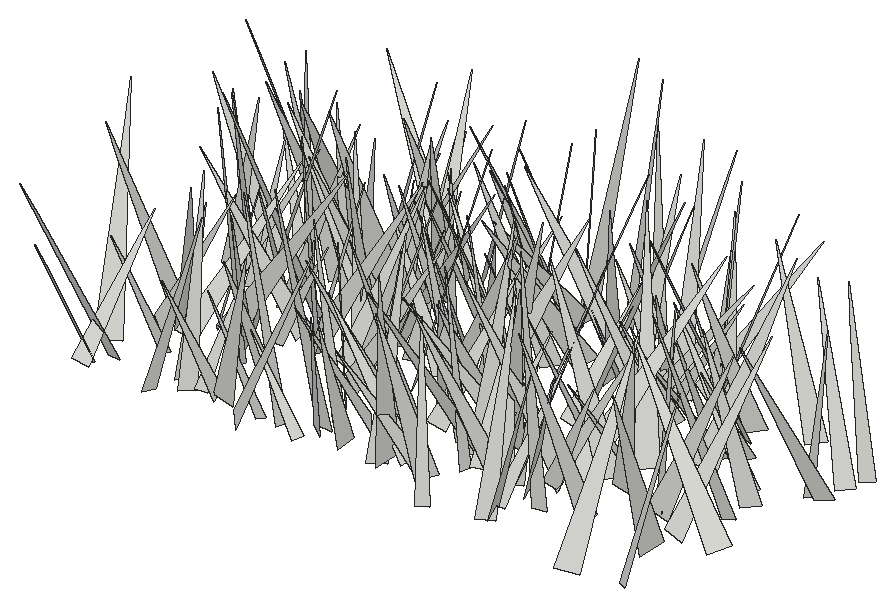
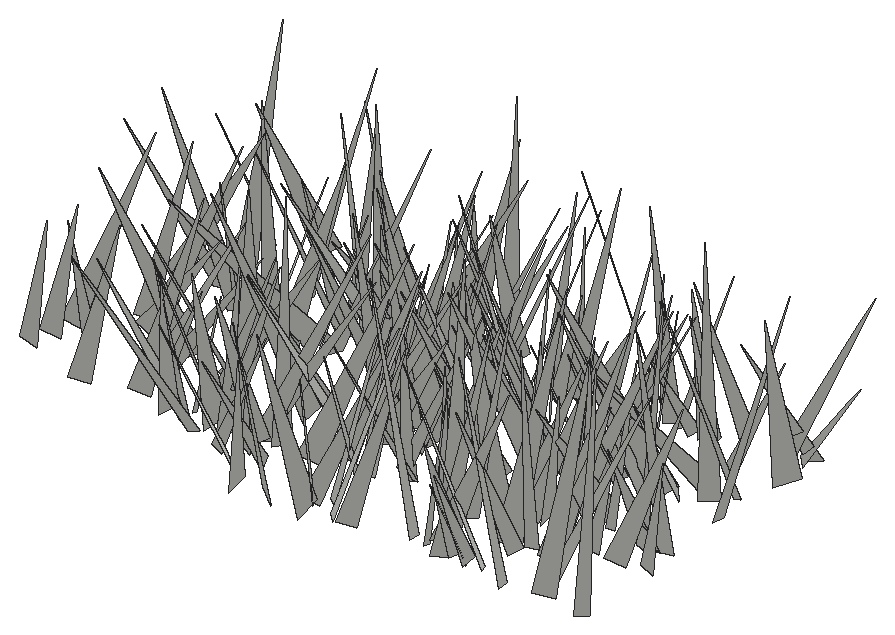
# SketchUp Ruby script. Lengths in inches.
U = 1.inch
M = Sketchup.active_model
def pt(a) = Geom::Point3d.new(a.map { |v| v * U })
def face(e, loops, mat)
  f = e.add_face(loops[0].map { |a| pt(a) })
  loops[1..].each { |l| e.add_face(l.map { |a| pt(a) }).erase! }
  f.material = f.back_material = mat if mat
  f
end
# faces: each face lists its corners as indices into pts; further lists are holes
def faces(e, pts, list, mat = nil) = list.each { |f| face(e, (f[0].is_a?(Array) ? f : [f]).map { |l| l.map { |i| pts[i] } }, mat) }
# xy, xz, yz: faces in a plane at the given z, y or x. An outline is a flat list of corners, or four numbers for a rectangle; further outlines are holes
def ring(l) = l.size == 4 ? [[l[0], l[1]], [l[2], l[1]], [l[2], l[3]], [l[0], l[3]]] : l.each_slice(2).to_a
def flat(e, list, mat, &to3) = list.each { |f| face(e, (f[0].is_a?(Array) ? f : [f]).map { |l| ring(l).map { |u, v| to3.(u, v) } }, mat) }
def xy(e, z, list, mat = nil) = flat(e, list, mat) { |x, y| [x, y, z] }
def xz(e, y, list, mat = nil) = flat(e, list, mat) { |x, z| [x, y, z] }
def yz(e, x, list, mat = nil) = flat(e, list, mat) { |y, z| [x, y, z] }
def lines(e, pts, list) = list.each { |a, b| e.add_line(pt(pts[a]), pt(pts[b])) }
# prism: a flat outline (further loops are holes) pulled along v
def prism(e, loops, v, mat = nil)
  f = face(e, loops, mat); d = Geom::Vector3d.new(v.map { |x| x * U })
  f.pushpull(f.normal.samedirection?(d) ? d.length : -d.length)
end
def box(e, o, s, mat = nil) = prism(e, [[o, [o[0] + s[0], o[1], o[2]], [o[0] + s[0], o[1] + s[1], o[2]], [o[0], o[1] + s[1], o[2]]]], [0, 0, s[2]], mat)
def at(x, y, z, deg = 0) = Geom::Transformation.translation(pt([x, y, z])) * Geom::Transformation.rotation(ORIGIN, Z_AXIS, deg.degrees)
def axes(o, x, y, z) = Geom::Transformation.new([*x, 0, *y, 0, *z, 0, *pt(o).to_a, 1])
def part(name) = M.definitions.add(name)
# library, detail: a bought-in or finely detailed component or shape, given as its bounding box
def library(name, o, s) = part(name).tap { |d| box(d.entities, o, s) }
def detail(e, o, s) = box(e.add_group.entities, o, s)
def put(e, d, t, mat = nil) = e.add_instance(d, t).tap { |i| i.material = mat if mat }
def group(e, t, mat = nil) = e.add_group.tap { |g| g.transformation = t; g.material = mat if mat }.entities
root = M.entities
c1 = part("fur_instance\#9")
p = [[0.8125,0,1.79],[0.67,-0.02,1.48],[0,-0.11,0],[0,0.11,0]]
faces(c1.entities,p,[[0,1,2,3]])
put(root,c1,axes([474.39,439.59,-21.66],[5.34642,-2.10558,1.0321],[-1.67954,-5.23165,-1.97278],[-1.63641,-1.50973,5.39684]))
put(root,c1,axes([480.85,439.32,-21.66],[4.14575,-5.15062,1.64406],[-4.88287,-4.45639,-1.64839],[-2.32151,0.17524,6.40304]))
put(root,c1,axes([477.65,439.58,-21.66],[7.83218,-2.47016,1.5817],[-2.12062,-7.88445,-1.81244],[-2.02643,-1.29626,8.00998]))
put(root,c1,axes([486.71,438.47,-21.66],[6.48852,0.93317,0.66882],[1.0636,-6.33108,-1.48501],[-0.43231,-1.57025,6.38486]))
put(root,c1,axes([464.62,439.47,-21.66],[-4.80536,-1.45342,1.08645],[-0.98448,4.67157,1.89512],[1.52434,-1.5647,4.64891]))
put(root,c1,axes([456.87,439.14,-21.66],[-2.83632,-6.0499,0.28173],[-5.90232,2.69141,-1.62612],[-1.35766,0.93829,6.48088]))
put(root,c1,axes([467.35,437.7,-21.66],[5.84897,4.9177,0.90335],[4.92852,-5.43629,-2.31659],[0.84231,-2.33947,7.282]))
put(root,c1,axes([465.28,439.13,-21.66],[0.87943,-6.58228,1.27772],[-6.45662,-0.48373,1.95201],[1.80858,1.47376,6.34739]))
put(root,c1,axes([496.97,440.95,-21.66],[6.98894,-3.62557,1.01436],[-3.15649,-6.80873,-2.58782],[-2.05189,-1.87497,7.43594]))
put(root,c1,axes([479.375,440.33,-21.66],[-5.28354,-0.86585,0.73138],[-0.45173,4.80676,2.42722],[1.0395,-2.31209,4.77222]))
put(root,c1,axes([456.21,437.95,-21.66],[-2.80536,-2.90649,0.0794],[-2.63209,2.49174,-1.78533],[-1.23535,1.29136,3.62358]))
put(root,c1,axes([471.7,438.33,-21.66],[-2.56697,2.61634,0.35758],[2.51502,2.27032,1.44317],[-0.80484,-1.25014,3.36925]))
put(root,c1,axes([482.8125,436.4375,-21.66],[0.07199,5.81915,0.58708],[5.58747,-0.24194,1.7129],[-1.72841,-0.53974,5.5618]))
put(root,c1,axes([472,439.81,-21.66],[-2.28168,-4.43341,1.38047],[-4.1851,2.6298,1.52839],[2.0114,0.44265,4.74608]))
put(root,c1,axes([492.07,441.03,-21.66],[-7.41474,-1.37074,2.09218],[-0.74138,7.45582,2.25736],[2.38883,-1.94072,7.19456]))
put(root,c1,axes([468.4375,438.84,-21.66],[-1.09532,-3.977,1.33167],[-3.82769,0.38536,-1.99748],[-1.71426,1.68065,3.6092]))
put(root,c1,axes([461.02,437.28,-21.66],[5.70541,0.17051,1.69377],[-0.31532,-5.71566,1.63753],[-1.67287,1.65887,5.46803]))
put(root,c1,axes([498.32,436.4,-21.66],[3.77258,4.9169,0.38845],[4.64704,-3.70729,1.79444],[-1.65279,0.7995,5.93196]))
put(root,c1,axes([494.63,435.64,-21.66],[-5.35866,5.61511,0.59327],[5.12673,5.1813,-2.73266],[2.36603,1.4904,7.2648]))
put(root,c1,axes([474.01,442.48,-21.66],[-4.88167,-3.98465,0.29136],[-3.56929,4.55624,2.50876],[1.79514,-1.77658,5.7805]))
put(root,c1,axes([478.73,440.36,-21.66],[-5.72955,1.74546,0.28048],[1.75274,5.48455,1.67353],[-0.23061,-1.68113,5.75097]))
put(root,c1,axes([455.63,437.38,-21.66],[-0.63862,5.35473,0.03552],[5.1577,0.62471,-1.44573],[1.43964,0.13724,5.19527]))
put(root,c1,axes([486.59,442.11,-21.66],[6.70588,0.95076,0.50826],[1.07552,-6.12086,-2.74035],[-0.07444,-2.78609,6.19381]))
put(root,c1,axes([472.22,440.24,-21.66],[1.71463,6.79892,3.94816],[7.36353,-2.80488,1.63226],[-2.7553,-3.26505,6.81916]))
put(root,c1,axes([469.95,439,-21.66],[-7.13799,-1.18277,0.6594],[-1.323,6.84565,-2.04241],[0.28881,2.12669,6.94107]))
put(root,c1,axes([486.875,437.47,-21.66],[-6.53703,2.92768,0.70077],[2.53956,6.26275,-2.47462],[1.61648,2.00045,6.72163]))
put(root,c1,axes([475.85,443.21,-21.66],[-6.75502,-2.37628,0.59319],[-2.11002,6.52988,2.13012],[1.24354,-1.82836,6.83664]))
put(root,c1,axes([481.92,443.48,-21.66],[-0.45254,-7.13046,0.09555],[-6.72101,0.39447,-2.39372],[-2.38342,0.24148,6.7319]))
put(root,c1,axes([458.82,441.61,-21.66],[-0.44719,-4.16584,0.88919],[-4.01944,0.11666,-1.47491],[-1.41032,0.98845,3.92158]))
put(root,c1,axes([462.83,438.76,-21.66],[-6.34351,2.24327,1.15963],[1.89857,6.30395,-1.80908],[1.66506,1.35834,6.48071]))
put(root,c1,axes([482.71,443.23,-21.66],[-6.34287,-0.8603,1.40577],[-0.30586,6.10717,2.3574],[1.61949,-2.21602,5.95103]))
put(root,c1,axes([463.48,439.26,-21.66],[-2.96386,2.60362,0.59977],[2.15648,2.85999,-1.75873],[1.5774,0.98217,3.53132]))
put(root,c1,axes([461.72,439.58,-21.66],[4.93577,0.48548,2.66433],[-0.37318,-5.36398,1.66873],[-2.68236,1.63958,4.67042]))
put(root,c1,axes([477.37,438.89,-21.66],[-6.45449,2.84921,1.13675],[2.42101,6.35763,-2.18855],[1.88385,1.59157,6.70736]))
put(root,c1,axes([464.63,443.83,-21.66],[4.72297,-1.05883,1.70864],[-0.28791,-4.67444,-2.10088],[-1.98939,-1.83725,4.36049]))
put(root,c1,axes([488.65,440.51,-21.66],[1.70019,7.5386,2.42367],[7.33263,-2.43467,2.42902],[-2.9895,-1.68439,7.33628]))
put(root,c1,axes([486.35,439.35,-21.66],[-3.43381,3.18637,0.41007],[2.54254,3.06224,-2.50406],[1.96382,1.60682,3.959]))
put(root,c1,axes([457.54,445.23,-21.66],[7.63705,-2.12328,0.08153],[-2.0044,-7.29978,-2.35267],[-0.70524,-2.24596,7.56953]))
put(root,c1,axes([487.33,443.23,-21.66],[1.64693,-4.65446,0.85777],[-4.4282,-1.19483,2.01879],[1.67056,1.42146,4.50564]))
put(root,c1,axes([482.33,445.56,-21.66],[2.66865,-7.95792,0.14871],[-7.80747,-2.5868,1.68053],[1.54726,0.67254,8.22351]))
put(root,c1,axes([482.03,441.6,-21.66],[-6.19983,-0.76734,1.02255],[-1.02443,6.01091,-1.70052],[0.76483,1.83095,6.01123]))
put(root,c1,axes([486.62,445.0625,-21.66],[-7.42366,-0.80204,0.92134],[-0.52005,7.2098,2.08597],[1.1053,-1.9946,7.16957]))
put(root,c1,axes([462.09,445.53,-21.66],[5.97611,0.87511,2.00016],[1.66713,-5.59279,-2.53411],[-1.40966,-2.90435,5.48252]))
put(root,c1,axes([472.375,441.51,-21.66],[0.67019,6.07953,1.22269],[5.42193,-1.17133,2.85227],[-3.0097,-0.75637,5.41058]))
put(root,c1,axes([476.1875,444.13,-21.66],[-1.63613,-6.00923,1.56488],[-6.02721,1.14742,-1.89548],[-1.49415,1.95172,5.93253]))
put(root,c1,axes([455.2,440.63,-21.66],[-6.50457,4.89284,0.5628],[4.72218,6.46057,-1.59001],[1.39918,0.94188,7.98255]))
put(root,c1,axes([491.06,445.6,-21.66],[0.69431,-7.1025,1.01226],[-6.95299,-0.41552,1.85354],[1.7681,1.15502,6.89145]))
put(root,c1,axes([500.24,443.42,-21.66],[-5.51381,4.9525,0.02994],[4.6746,5.18943,2.47955],[-1.63592,-1.86355,6.98435]))
put(root,c1,axes([481.2,446.75,-21.66],[-6.30471,-1.37126,0.42808],[-1.05468,5.72683,2.8114],[0.97532,-2.67133,5.80738]))
put(root,c1,axes([456.37,444.01,-21.66],[3.98085,5.13777,1.04709],[4.9615,-3.26572,-2.83883],[1.69606,-2.50573,5.84679]))
put(root,c1,axes([485.77,442.15,-21.66],[-3.80527,0.70423,0.62745],[0.3357,3.44844,-1.83447],[0.88144,1.72686,3.40746]))
put(root,c1,axes([487.24,443.55,-21.66],[3.70489,5.29932,0.63458],[5.07029,-3.25343,-2.43293],[1.66665,-1.88258,5.99082]))
put(root,c1,axes([484.94,441.74,-21.66],[-5.93651,2.05948,0.4431],[1.83167,5.70073,-1.95618],[1.04056,1.71471,5.97135]))
put(root,c1,axes([490.35,447.48,-21.66],[-3.99829,-3.957,0.07334],[-3.50173,3.58563,2.55553],[1.84422,-1.77059,5.01133]))
put(root,c1,axes([480.05,444.08,-21.66],[-1.59145,-6.67923,2.98055],[-7.18236,0.85085,-1.92829],[-1.38185,3.26993,6.58988]))
put(root,c1,axes([471.7,442.98,-21.66],[-4.19914,-2.372,1.71601],[-2.90919,3.71707,-1.98087],[0.32817,2.60017,4.39719]))
put(root,c1,axes([455.65,446.73,-21.66],[-7.05336,-2.15617,1.71578],[-1.62887,7.06566,2.18314],[2.22256,-1.66441,7.04506]))
put(root,c1,axes([494.52,444.51,-21.66],[2.05152,-6.6713,2.37008],[-6.64568,-0.96384,3.03943],[2.44098,2.98279,6.28306]))
put(root,c1,axes([482.3,443.26,-21.66],[0.05703,4.78722,0.58826],[4.57544,0.13244,-1.52137],[1.52606,-0.57598,4.5394]))
put(root,c1,axes([482.55,442.21,-21.66],[-4.05374,2.9207,0.15477],[2.65047,3.78022,-1.91631],[1.23673,1.47198,4.61422]))
put(root,c1,axes([479.28,447.84,-21.66],[5.03177,-2.92165,1.14225],[-2.20313,-4.82824,-2.64459],[-2.23316,-1.81978,5.18275]))
put(root,c1,axes([475.85,447.31,-21.66],[5.48383,-1.63022,0.30334],[-1.45467,-5.23263,-1.82362],[-0.79597,-1.66854,5.42259]))
put(root,c1,axes([470.08,445.46,-21.66],[3.77376,6.10396,1.49671],[5.76595,-2.66802,-3.65722],[2.50047,-3.05991,6.17449]))
put(root,c1,axes([463.42,443.4,-21.66],[-7.24108,-2.76695,1.69952],[-3.23599,6.49389,-3.21487],[0.2698,3.62643,7.05364]))
put(root,c1,axes([496.91,443.12,-21.66],[1.06363,7.1406,0.14161],[6.98782,-1.01087,-1.51263],[1.47601,-0.35985,7.05914]))
put(root,c1,axes([485.63,441.875,-21.66],[6.81061,4.1437,0.72104],[3.52808,-6.3754,3.31382],[-2.28972,2.50169,7.25074]))
put(root,c1,axes([481.43,443.62,-21.66],[-6.63675,3.07759,1.929],[2.57186,6.8191,-2.03087],[2.56478,1.12578,7.02806]))
put(root,c1,axes([470.89,445.98,-21.66],[7.00496,3.81978,0.96353],[3.93839,-6.83549,-1.53416],[-0.09034,-1.80938,7.82984]))
put(root,c1,axes([489.6,446.23,-21.66],[-4.16416,5.80884,2.0419],[6.1268,3.66414,2.07088],[-0.6118,-2.84317,6.84063]))
put(root,c1,axes([477.32,444.6875,-21.66],[-0.99691,5.86129,1.26655],[5.41282,1.43213,-2.36709],[2.58075,-0.73958,5.45394]))
put(root,c1,axes([498.29,446.77,-21.66],[-2.5015,-6.23633,1.72664],[-6.18785,1.76379,-2.59425],[-1.89304,2.47545,6.19832]))
put(root,c1,axes([463.37,446.58,-21.66],[3.09859,-2.8989,0.71648],[-2.92503,-2.73871,1.56906],[0.60101,1.61681,3.94246]))
put(root,c1,axes([485.45,449.1875,-21.66],[-4.40501,-3.46188,0.56585],[-3.18391,4.32713,1.68747],[1.47225,-1.00011,5.34239]))
put(root,c1,axes([460.18,446.09,-21.66],[5.69226,-5.26322,0.96159],[-5.00885,-4.7486,3.65927],[1.88086,3.28288,6.8347]))
put(root,c1,axes([463.9,448.61,-21.66],[-7.08449,-0.21202,0.14595],[-0.16992,6.87165,1.73429],[0.19334,-1.72965,6.8722]))
put(root,c1,axes([494.42,444.8,-21.66],[3.23969,5.31398,1.47982],[4.81259,-3.56155,2.25346],[-2.69577,0.02794,5.80137]))
put(root,c1,axes([469.3,447.15,-21.66],[1.72384,-3.5656,0.8716],[-3.29525,-1.07913,2.10276],[1.61693,1.60212,3.35612]))
put(root,c1,axes([458.59,443.9,-21.66],[-3.50989,5.55769,0.51718],[4.45011,3.15505,-3.70364],[3.36927,1.62248,5.4305]))
put(root,c1,axes([498.33,448.82,-21.66],[-3.08305,4.83073,2.80211],[5.58378,2.72141,1.452],[0.09585,-3.15451,5.54372]))
put(root,c1,axes([459.51,445.8,-21.66],[3.36886,3.17868,0.5186],[2.75759,-3.23451,1.91201],[-1.66392,1.0752,4.2187]))
put(root,c1,axes([475.19,449.19,-21.66],[4.73655,-6.32836,0.37656],[-6.13582,-4.45802,2.25891],[1.59428,1.644,7.57499]))
put(root,c1,axes([477.25,449.4,-21.66],[0.83878,-6.84447,1.51714],[-6.71971,-0.34936,2.13903],[1.99848,1.69801,6.55552]))
put(root,c1,axes([474.93,450.21,-21.66],[-7.14717,-1.7401,1.8273],[-1.33254,7.26397,1.70532],[2.14274,-1.28679,7.15555]))
put(root,c1,axes([479.69,447.47,-21.66],[-6.30755,-1.0303,0.95825],[-1.23667,6.15876,-1.51833],[0.67114,1.66527,6.20817]))
put(root,c1,axes([481.65,447.47,-21.66],[-4.16837,-0.36819,0.02902],[-0.35612,3.91965,-1.4217],[-0.09791,1.41863,3.93569]))
put(root,c1,axes([466.52,445.98,-21.66],[3.68113,4.53912,0.36663],[4.24955,-3.59341,1.82137],[-1.63686,0.87892,5.5531]))
put(root,c1,axes([468.27,447.03,-21.66],[1.11802,6.55656,0.88639],[6.4324,-0.86675,-1.70208],[1.54866,-1.13332,6.42972]))
put(root,c1,axes([471.41,446.45,-21.66],[4.34106,2.99141,0.28027],[2.79242,-4.19877,1.56351],[-1.10882,1.13738,5.03476]))
put(root,c1,axes([464.87,449.39,-21.66],[4.40787,6.56573,1.54887],[6.23945,-3.26461,-3.91775],[2.5646,-3.34225,6.86945]))
put(root,c1,axes([471.2,446.76,-21.66],[4.43621,4.25023,1.48293],[3.65379,-4.61591,2.29927],[-2.62932,0.75659,5.69717]))
put(root,c1,axes([466.13,447.23,-21.66],[-6.09623,-2.24198,1.5344],[-2.70516,5.35755,-2.91953],[0.25098,3.28863,5.80232]))
put(root,c1,axes([487.96,444.86,-21.66],[-4.06981,7.2471,0.38585],[5.9474,3.58401,-4.58433],[4.15906,1.9665,6.9331]))
put(root,c1,axes([460.03,451.74,-21.66],[-1.799,-4.93024,0.4482],[-4.7112,1.85147,1.45641],[1.52075,-0.09654,5.04207]))
put(root,c1,axes([463.41,450.76,-21.66],[-3.74944,-6.99723,1.04952],[-6.92154,3.38084,-2.18706],[-1.468,1.93125,7.63127]))
put(root,c1,axes([501.3,452.24,-21.66],[1.05272,-6.58483,0.46236],[-6.33643,-1.13928,-1.79827],[-1.85027,0.15508,6.42141]))
put(root,c1,axes([473.59,449.86,-21.66],[-3.5373,3.73043,1.14853],[3.88761,3.22863,1.48666],[-0.34887,-1.84596,4.92122]))
put(root,c1,axes([461.47,446.71,-21.66],[6.96857,3.90701,1.2479],[3.36407,-6.85211,2.66731],[-2.34628,1.77954,7.53068]))
put(root,c1,axes([466.48,451.89,-21.66],[6.75782,0.35235,2.65885],[1.16075,-6.88187,-2.03823],[-2.41791,-2.31896,6.45275]))
put(root,c1,axes([473.24,447.58,-21.66],[6.6915,4.26773,1.20587],[3.94044,-6.72308,1.92792],[-2.03484,1.01512,7.69888]))
put(root,c1,axes([457.08,452.37,-21.66],[-3.46246,-6.72611,1.90114],[-6.59046,3.84836,1.61233],[2.32826,0.89059,7.39118]))
put(root,c1,axes([477.18,451.99,-21.66],[2.07111,-6.85146,1.31632],[-6.80663,-1.68294,1.94991],[1.53132,1.78604,6.88693]))
put(root,c1,axes([493.41,452.37,-21.66],[-0.91918,-4.72146,0.08029],[-4.18667,0.777,-2.23865],[-2.18412,0.49761,4.25741]))
put(root,c1,axes([479.12,451.43,-21.66],[-4.75874,-5.64309,0.42264],[-5.39038,4.3522,-2.58279],[-1.72245,1.97043,6.91515]))
put(root,c1,axes([475.43,450.9,-21.66],[-3.98273,-4.40716,0.90523],[-4.3967,3.55588,-2.0321],[-0.95477,2.0093,5.58174]))
put(root,c1,axes([494.61,453.16,-21.66],[2.5877,-3.76016,0.15432],[-3.53923,-2.49522,-1.45139],[-1.27925,-0.70276,4.32764]))
put(root,c1,axes([490.53,448.49,-21.66],[-7.32021,3.8589,0.48336],[3.73123,7.2592,-1.44642],[1.09666,1.05977,8.14767]))
put(root,c1,axes([497.41,450.02,-21.66],[-2.18408,5.95276,0.46734],[5.01759,1.55993,3.57972],[-3.2369,-1.59851,5.23366]))
put(root,c1,axes([477.19,450.11,-21.66],[0.42432,7.03314,2.02201],[6.63788,0.48281,-3.07232],[3.08094,-2.00885,6.34082]))
put(root,c1,axes([455.55,452,-21.66],[-0.42435,-6.57592,2.54627],[-6.78158,1.0798,1.65847],[1.93298,2.34469,6.37748]))
put(root,c1,axes([467.35,449.82,-21.66],[0.02975,6.47261,1.15989],[6.34372,-0.33363,1.69906],[-1.73125,-1.11127,6.2457]))
put(root,c1,axes([468.71,448.12,-21.66],[7.42059,-0.17453,3.00871],[-1.57677,-7.03899,3.48057],[-2.56838,3.81708,6.55601]))
put(root,c1,axes([489.61,451.72,-21.66],[-2.20634,6.02099,1.75888],[5.48729,0.94934,3.63349],[-3.03901,-2.65713,5.28374]))
put(root,c1,axes([469.09,450.8125,-21.66],[6.564,-1.73993,0.0582],[-1.67851,-6.26496,2.01239],[0.46191,1.95953,6.48565]))
put(root,c1,axes([488.56,453.96,-21.66],[3.46257,-3.0651,1.27719],[-2.41097,-3.5895,-2.07802],[-2.28326,-0.85797,4.13111]))
put(root,c1,axes([483.36,449.92,-21.66],[-0.37436,5.47936,0.25355],[5.20879,0.43477,-1.70506],[1.71934,-0.12411,5.22075]))
put(root,c1,axes([477.8,451.14,-21.66],[-2.08516,6.03207,0.25096],[5.29839,1.7011,3.1353],[-2.89412,-1.23172,5.5591]))
put(root,c1,axes([465.28,454.17,-21.66],[1.50286,-5.49819,1.33251],[-5.18917,-1.88889,-1.94134],[-2.25347,0.68284,5.35909]))
put(root,c1,axes([471.03,449.97,-21.66],[-4.89219,1.92037,1.37183],[1.09822,4.64707,-2.5888],[2.08893,2.05431,4.57377]))
put(root,c1,axes([479.55,456.4,-21.66],[4.2838,-6.03866,0.74714],[-5.20831,-4.11147,-3.36808],[-3.14598,-1.41597,6.59337]))
put(root,c1,axes([456.18,452,-21.66],[3.26284,4.45559,0.15103],[4.26787,-3.06768,-1.7017],[1.28856,-1.1217,5.25381]))
put(root,c1,axes([473.22,454.7,-21.66],[5.22724,-1.35677,0.09683],[-1.28473,-5.05093,-1.4184],[-0.44684,-1.34966,5.21086]))
put(root,c1,axes([493.1,450.8125,-21.66],[-3.36255,6.42423,2.20976],[5.77924,4.00105,-2.8377],[3.57129,-0.42595,6.67271]))
put(root,c1,axes([464.39,454.2,-21.66],[-6.62778,2.24684,1.33683],[2.5489,6.36376,1.94128],[0.58185,-2.2841,6.72363]))
put(root,c1,axes([467.13,453.58,-21.66],[2.95876,-6.29379,1.88961],[-6.54545,-2.63888,1.45948],[0.58268,2.31543,6.79971]))
put(root,c1,axes([467.43,455.76,-21.66],[6.21031,-0.46369,2.15458],[0.49806,-5.98034,-2.72263],[-2.14689,-2.7287,5.60092]))
put(root,c1,axes([474.2,454.09,-21.66],[-1.75901,-5.06572,0.78099],[-4.97011,1.48393,-1.5689],[-1.25276,1.22556,5.12778]))
put(root,c1,axes([475.41,455.64,-21.66],[-2.3415,-4.6423,0.1365],[-4.37976,2.25803,1.66471],[1.54509,-0.63449,4.92568]))
put(root,c1,axes([482.94,451.9375,-21.66],[8.11647,0.24258,0.67526],[0.10402,-7.98511,1.61836],[-0.70993,1.60345,7.95719]))
put(root,c1,axes([461.125,450.19,-21.66],[-5.44791,2.04028,1.98238],[0.64646,5.0587,-3.42987],[2.77031,2.83181,4.69878]))
put(root,c1,axes([457.88,451.11,-21.66],[-4.70225,1.57903,0.9136],[0.9953,4.33742,-2.37389],[1.52885,2.03289,4.35536]))
put(root,c1,axes([500.39,451.84,-21.66],[-4.99347,0.21503,1.45697],[-0.36457,4.80955,-1.95935],[1.42691,1.98134,4.59803]))
put(root,c1,axes([463.8,456.93,-21.66],[5.79186,-5.56058,1.06137],[-5.14067,-5.80215,-2.34538],[-2.37068,-1.00358,7.67886]))
put(root,c1,axes([478.11,454.79,-21.66],[1.0703,-6.74535,2.51722],[-6.58595,-1.94546,-2.41292],[-2.90886,1.9228,6.3893]))
put(root,c1,axes([461.73,451.96,-21.66],[2.76553,6.92914,2.18566],[6.51494,-3.40021,2.53621],[-3.21647,-0.92942,7.01632]))
put(root,c1,axes([481.97,456.03,-21.66],[7.49694,-1.26912,1.50095],[-0.87324,-7.45265,-1.93987],[-1.76095,-1.70734,7.35199]))
put(root,c1,axes([493.17,454.98,-21.66],[-4.54236,-5.48641,0.31776],[-5.31376,4.27953,-2.06985],[-1.40202,1.55551,6.81539]))
put(root,c1,axes([457.25,454.74,-21.66],[-3.27496,5.22829,1.96451],[5.47571,2.5569,2.32348],[-1.10043,-2.83671,5.71505]))
put(root,c1,axes([460.53,456.96,-21.66],[0.98136,-7.62341,0.77855],[-7.49654,-1.11781,-1.49599],[-1.58884,0.56543,7.53933]))
put(root,c1,axes([468.05,457.01,-21.66],[0.34985,-8.1007,0.677],[-7.9597,-0.20383,1.67442],[1.6501,0.73429,7.93347]))
put(root,c1,axes([492.8,456.26,-21.66],[2.20766,-6.15742,1.48059],[-5.96151,-2.54967,-1.71445],[-2.13691,0.75174,6.31254]))
put(root,c1,axes([483.37,456.4,-21.66],[-7.87957,1.88276,1.17896],[2.17634,7.41366,2.70618],[0.44527,-2.91806,7.63603]))
put(root,c1,axes([486.42,455.83,-21.66],[-4.94323,1.53486,1.76986],[2.06825,4.80019,1.61379],[1.10026,-2.12747,4.91803]))
put(root,c1,axes([488.65,456.1,-21.66],[-3.02452,-1.82217,1.01563],[-1.34667,3.07159,1.50047],[1.5932,-0.86291,3.19635]))
put(root,c1,axes([485.88,454.07,-21.66],[4.06376,5.39951,0.02576],[4.83357,-3.62337,-3.0294],[2.40665,-1.8401,6.04083]))
put(root,c1,axes([463.83,453.02,-21.66],[-6.21207,0.31771,0.7174],[0.09871,5.99609,-1.80072],[0.77837,1.77522,5.95384]))
put(root,c1,axes([485.68,456.9,-21.66],[4.75134,-2.11282,0.36953],[-1.90852,-4.57438,-1.61505],[-0.97883,-1.33672,4.94275]))
put(root,c1,axes([471.47,453.53,-21.66],[-5.20455,-0.25594,1.25726],[-0.61037,5.11409,-1.48563],[1.12857,1.58561,4.99457]))
put(root,c1,axes([492.19,454.92,-21.66],[0.25275,3.74041,1.98428],[3.79537,-1.08135,1.55493],[-1.87703,-1.68284,3.41127]))
put(root,c1,axes([484.07,454.69,-21.66],[-5.6206,-6.05261,0.8091],[-5.56666,4.62654,-4.06048],[-2.5102,3.29256,7.1929]))
put(root,c1,axes([462.26,456.52,-21.66],[-0.76172,-5.93829,1.58025],[-5.83151,1.20063,1.7008],[1.93753,1.27903,5.74028]))
put(root,c1,axes([455.15,454.27,-21.66],[0.45308,4.94253,1.25959],[4.74966,-0.86975,1.70432],[-1.859,-1.01755,4.66145]))
put(root,c1,axes([501.5,454.01,-21.66],[-1.94953,6.2532,0.70862],[6.08536,1.68405,1.8809],[-1.60411,-1.2111,6.27419]))
put(root,c1,axes([459.29,454.49,-21.66],[-1.35626,4.67986,0.4324],[4.48876,1.15652,1.56235],[-1.3925,-0.82998,4.61514]))
put(root,c1,axes([486.68,456.09,-21.66],[3.67258,4.04026,0.63824],[3.75616,-2.99162,-2.6759],[1.61937,-2.22383,4.75932]))
put(root,c1,axes([473.07,454.44,-21.66],[2.06268,4.77096,0.10661],[4.57909,-1.94603,-1.50762],[1.34363,-0.69206,4.97431]))
put(root,c1,axes([479.83,452.55,-21.66],[6.02604,4.35688,0.13616],[4.14402,-5.7981,2.12678],[-1.35204,1.64734,7.12547]))
put(root,c1,axes([461.44,454.82,-21.66],[0.20171,6.63601,2.13173],[6.14884,-1.17367,3.07178],[-3.28217,-1.79094,5.8857]))
put(root,c1,axes([458.05,460.59,-21.66],[7.18044,-3.7228,0.21814],[-3.29243,-6.55088,-3.42221],[-1.75122,-2.94828,7.32847]))
put(root,c1,axes([476.39,460.25,-21.66],[3.78174,-4.82109,0.17581],[-4.12071,-3.34423,-3.06777],[-2.50869,-1.77444,5.30408]))
put(root,c1,axes([501.91,455.6,-21.66],[-0.60049,6.11637,0.8715],[5.86899,0.29123,2.00004],[-1.92986,-1.0175,5.81123]))
put(root,c1,axes([475.22,459.57,-21.66],[-4.26482,-5.03014,0.77761],[-4.82923,4.31941,1.45497],[1.60794,-0.36894,6.43227]))
put(root,c1,axes([473.72,459.23,-21.66],[-3.75985,-4.2409,1.14983],[-3.97997,3.92819,1.47409],[1.86202,-0.16705,5.47255]))
put(root,c1,axes([459.25,457.78,-21.66],[-5.59942,-5.49473,0.70955],[-5.42162,5.22657,-2.3104],[-1.14084,2.13071,7.49717]))
put(root,c1,axes([454.72,461.07,-21.66],[-1.50636,-7.45489,0.25307],[-6.77182,1.47502,3.14252],[3.12761,-0.39686,6.92598]))
put(root,c1,axes([474.0625,461.05,-21.66],[-5.99255,-5.60768,0.41861],[-5.37957,5.89507,1.95969],[1.63755,-1.155,7.96972]))
put(root,c1,axes([496.56,457.36,-21.66],[-3.37701,5.49526,1.43426],[5.6473,3.0721,1.52623],[-0.60248,-2.00587,6.26679]))
put(root,c1,axes([465.97,460.81,-21.66],[6.61822,-2.56323,1.80089],[-1.74555,-6.51281,-2.85492],[-2.60123,-2.15113,6.49773]))
put(root,c1,axes([462.75,457.43,-21.66],[4.25693,-2.37845,0.80532],[-2.50825,-3.95225,1.586],[0.11926,1.77474,4.61119]))
put(root,c1,axes([484.76,458.8,-21.66],[-1.35927,-4.19334,1.10265],[-4.18909,0.97193,-1.4678],[-1.11869,1.45561,4.1566]))
put(root,c1,axes([468.66,459.88,-21.66],[7.66511,2.45698,1.17946],[2.70747,-7.26796,-2.45522],[-0.3122,-2.70587,7.66567]))
put(root,c1,axes([467.47,460.13,-21.66],[-4.01189,-2.17426,1.82805],[-1.57492,4.33524,1.69992],[2.36407,-0.80168,4.23473]))
put(root,c1,axes([490.02,456.9,-21.66],[-5.70534,2.42628,0.74712],[2.22137,5.6608,-1.42016],[1.22905,1.03174,6.03498]))
put(root,c1,axes([489.1875,456.41,-21.66],[2.9038,6.51052,1.10748],[6.2299,-3.10193,1.9005],[-2.1913,-0.1914,6.87074]))
put(root,c1,axes([483.26,456.625,-21.66],[-5.22484,3.83291,1.4033],[3.4058,5.3502,-1.93269],[2.24967,0.80218,6.18505]))
put(root,c1,axes([472.83,461.23,-21.66],[2.63198,-5.20128,0.6124],[-4.94839,-2.69423,-1.6156],[-1.71515,-0.20845,5.60093]))
put(root,c1,axes([489.37,456.49,-21.66],[5.91646,3.40669,0.5347],[3.12979,-5.75065,2.00759],[-1.44773,1.49011,6.52531]))
put(root,c1,axes([475.08,457.04,-21.66],[4.44395,3.96646,1.43413],[3.47391,-4.62357,2.02305],[-2.39195,0.65422,5.60257]))
put(root,c1,axes([486.83,456.36,-21.66],[-7.37463,3.18086,0.67882],[2.84062,7.11825,-2.49505],[1.58417,2.04365,7.63399]))
put(root,c1,axes([483.39,457.81,-21.66],[0.65103,4.23875,0.31259],[3.78552,-0.72206,1.9071],[-1.9325,0.01355,3.84107]))
put(root,c1,axes([487.25,457.93,-21.66],[2.23337,6.49328,0.05356],[5.9184,-2.0122,-2.84202],[2.67172,-0.9705,6.25089]))
put(root,c1,axes([462.99,460.29,-21.66],[5.8637,3.4963,0.04079],[3.31459,-5.53283,-2.23832],[1.11324,-1.94227,6.44958]))
put(root,c1,axes([466.95,459.23,-21.66],[-5.54363,5.04114,0.10568],[4.92423,5.3789,1.72499],[-1.08457,-1.34553,7.29173]))
put(root,c1,axes([460.75,461.22,-21.66],[6.83601,2.20523,1.02382],[2.40175,-6.59991,-1.82073],[-0.37792,-2.05437,6.94831]))
put(root,c1,axes([481.4,458.42,-21.66],[4.67368,1.9817,0.84614],[1.46066,-4.3994,2.23565],[-1.58416,1.79011,4.55767]))
put(root,c1,axes([476.51,459.85,-21.66],[3.82585,4.29132,1.89582],[3.55577,-4.24822,2.44044],[-3.06039,0.42878,5.20545]))
put(root,c1,axes([464.22,460.13,-21.66],[-4.08665,1.67614,0.95166],[1.15635,3.91687,-1.93308],[1.54207,1.50482,3.97156]))
put(root,c1,axes([464.62,460.18,-21.66],[2.09645,3.63188,0.13416],[3.39461,-2.01213,1.42535],[-1.29816,0.60366,3.94386]))
put(root,c1,axes([483.36,459.36,-21.66],[4.16098,5.56887,0.17793],[5.30628,-4.02846,1.99315],[-1.69922,1.05685,6.65984]))
put(root,c1,axes([465.27,459.74,-21.66],[-4.827,3.94667,0.05385],[3.76525,4.62978,-1.80751],[1.18405,1.36675,5.96733]))
put(root,c1,axes([481.06,461.5,-21.66],[-6.67208,0.88571,0.68005],[0.61302,6.34873,-2.25421],[0.93335,2.16166,6.3419]))
put(root,c1,axes([478.76,461.53,-21.66],[4.06044,6.49572,1.60929],[6.19974,-4.35997,1.95581],[-2.5194,-0.26008,7.4065]))
put(root,c1,axes([475.8,461.25,-21.66],[7.23662,0.86237,3.59764],[-0.54989,-7.56504,2.91946],[-3.65846,2.84288,6.67751]))
